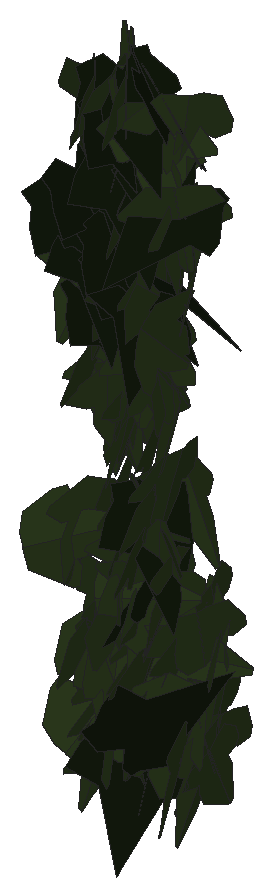
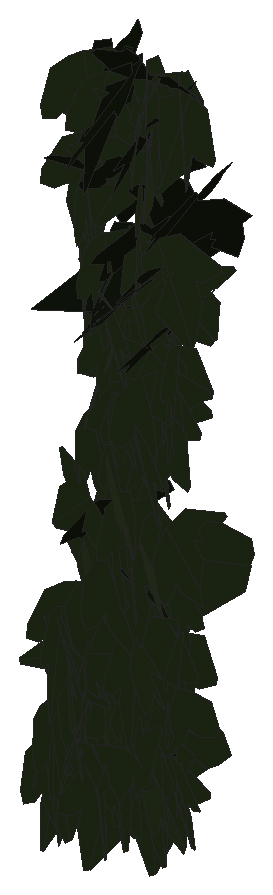
# SketchUp Ruby script. Lengths in inches.
U = 1.inch
M = Sketchup.active_model
def pt(a) = Geom::Point3d.new(a.map { |v| v * U })
def face(e, loops, mat)
  f = e.add_face(loops[0].map { |a| pt(a) })
  loops[1..].each { |l| e.add_face(l.map { |a| pt(a) }).erase! }
  f.material = f.back_material = mat if mat
  f
end
# faces: each face lists its corners as indices into pts; further lists are holes
def faces(e, pts, list, mat = nil) = list.each { |f| face(e, (f[0].is_a?(Array) ? f : [f]).map { |l| l.map { |i| pts[i] } }, mat) }
# xy, xz, yz: faces in a plane at the given z, y or x. An outline is a flat list of corners, or four numbers for a rectangle; further outlines are holes
def ring(l) = l.size == 4 ? [[l[0], l[1]], [l[2], l[1]], [l[2], l[3]], [l[0], l[3]]] : l.each_slice(2).to_a
def flat(e, list, mat, &to3) = list.each { |f| face(e, (f[0].is_a?(Array) ? f : [f]).map { |l| ring(l).map { |u, v| to3.(u, v) } }, mat) }
def xy(e, z, list, mat = nil) = flat(e, list, mat) { |x, y| [x, y, z] }
def xz(e, y, list, mat = nil) = flat(e, list, mat) { |x, z| [x, y, z] }
def yz(e, x, list, mat = nil) = flat(e, list, mat) { |y, z| [x, y, z] }
def lines(e, pts, list) = list.each { |a, b| e.add_line(pt(pts[a]), pt(pts[b])) }
# prism: a flat outline (further loops are holes) pulled along v
def prism(e, loops, v, mat = nil)
  f = face(e, loops, mat); d = Geom::Vector3d.new(v.map { |x| x * U })
  f.pushpull(f.normal.samedirection?(d) ? d.length : -d.length)
end
def box(e, o, s, mat = nil) = prism(e, [[o, [o[0] + s[0], o[1], o[2]], [o[0] + s[0], o[1] + s[1], o[2]], [o[0], o[1] + s[1], o[2]]]], [0, 0, s[2]], mat)
def at(x, y, z, deg = 0) = Geom::Transformation.translation(pt([x, y, z])) * Geom::Transformation.rotation(ORIGIN, Z_AXIS, deg.degrees)
def axes(o, x, y, z) = Geom::Transformation.new([*x, 0, *y, 0, *z, 0, *pt(o).to_a, 1])
def part(name) = M.definitions.add(name)
# library, detail: a bought-in or finely detailed component or shape, given as its bounding box
def library(name, o, s) = part(name).tap { |d| box(d.entities, o, s) }
def detail(e, o, s) = box(e.add_group.entities, o, s)
def put(e, d, t, mat = nil) = e.add_instance(d, t).tap { |i| i.material = mat if mat }
def group(e, t, mat = nil) = e.add_group.tap { |g| g.transformation = t; g.material = mat if mat }.entities
root = M.entities
M.materials.add("efeu1").color = [18, 25, 13]
M.materials.add("efeu2").color = [43, 57, 29]
c1 = part("ivyleaf_10")
p = [[0,0.5,-0.03],[-0.0625,2.02,-0.43],[-0.19,2.01,-0.46],[-0.54,1.05,-0.29],[-0.52,0.625,-0.18],[-0.83,0.76,-0.28],
  [-1.16,0.64,-0.33],[-1.15,0.33,-0.24],[-0.77,-0.39,0.02],[-0.3,-0.51,0.16],[0.04,-0.48,0.23],[-0.02,2.01,-0.4375],
  [-0.06,2.01,-0.43],[0.04,-0.49,0.23],[0.67,-0.49,0.14],[1.38,0.36,-0.2],[1.375,0.51,-0.24],[0.81,0.65,-0.19],
  [0.62,0.59,-0.15],[0.6,1.09,-0.28],[0.5,1.23,-0.31]]
faces(c1.entities,p,[[0,1,2,3,4,5,6,7,8,9,10],[11,12,0,13,14,15,16,17,18,19,20]],"efeu2")
c2 = part("ivyleaf_9")
p = [[1.54,2.16,1.25],[1.36,2.04,1.19],[-0.21,0.99,0.68],[-0.71,1.11,0.82],[-0.85,0.86,0.67],[-0.8,0.17,0.21],
  [-0.9,-0.01,0.1],[-0.67,-0.16,-0.02],[-0.08,-0.08,-0.05],[-0.03,-0.6,-0.4],[0.65,-0.88,-0.66],[0.83,-0.6,-0.49],
  [1.29,-0.42,-0.43],[1.8125,-0.07,-0.26],[1.21,0.44,0.15]]
faces(c2.entities,p,[[0,1,2,3,4,5,6,7,8,9,10,11,12,13,14]],"efeu1")
put(root,c1,axes([19.25,224.81,220.86],[-0.42384,-0.16044,0.21122],[-0.18486,-0.10687,-0.45211],[0.19022,-0.46134,0.03127]))
put(root,c1,axes([19.05,224.78,217.3],[-0.02524,-0.43944,0.23719],[0.06704,-0.23832,-0.43441],[0.49484,0.00987,0.07095]))
put(root,c1,axes([19.06,225.11,214.47],[0.12032,-0.4664,0.13412],[0.03183,-0.1303,-0.48167],[0.48426,0.12445,-0.00167]))
put(root,c1,axes([18.77,224.23,216.92],[0.07583,0.04521,-0.49214],[0.42938,0.2405,0.08825],[0.2447,-0.43602,-0.00235]))
put(root,c1,axes([19.11,224.54,215.75],[0.05155,-0.43916,-0.23342],[0.04918,0.23802,-0.43695],[0.4949,0.02209,0.06774]))
put(root,c1,axes([19.14,224.71,220.44],[-0.21372,-0.34408,0.29314],[0.05065,-0.34044,-0.36267],[0.44918,-0.12532,0.18037]))
put(root,c1,axes([19.35,224.875,214.3],[-0.36082,0.16197,0.30589],[-0.29662,0.08304,-0.39385],[-0.17839,-0.46569,0.03616]))
put(root,c1,axes([19.12,224.66,222.71],[-0.4928,0.05479,-0.06441],[0.06274,-0.01843,-0.49571],[-0.0567,-0.49665,0.01129]))
put(root,c1,axes([18.9375,224.98,215.45],[0.43453,0.18103,0.16855],[0.15335,0.07018,-0.4707],[-0.19408,0.46076,0.00546]))
put(root,c1,axes([19.1875,224.95,214.75],[-0.00417,-0.49987,-0.01051],[0.00087,0.0105,-0.49989],[0.49998,-0.00419,0.00078]))
put(root,c1,axes([19.2,224.53,219.39],[0.04854,-0.43156,-0.24778],[-0.01141,0.24793,-0.43405],[0.49751,0.04779,0.01422]))
put(root,c1,axes([19.2,225.08,215.99],[0.07684,-0.45309,0.19698],[0.02088,-0.19619,-0.45943],[0.49362,0.07883,-0.01123]))
put(root,c1,axes([19.22,224.67,214.375],[0.39934,-0.29803,-0.04127],[-0.0295,0.02947,-0.49826],[0.29942,0.40039,0.00595]))
put(root,c1,axes([19.24,224.42,222.76],[0.21719,-0.434,-0.12029],[0.00579,0.13623,-0.48105],[0.45033,0.20756,0.0642]))
put(root,c1,axes([19.28,224.93,214.23],[-0.18051,-0.46447,-0.04109],[0.00929,0.04047,-0.49827],[0.46619,-0.18065,-0.00599]))
put(root,c1,axes([19.1,225.21,217.36],[0.24568,-0.33864,0.2738],[0.18002,-0.20727,-0.41789],[0.39653,0.30391,0.02008]))
put(root,c1,axes([19.19,224.91,218.74],[-0.46671,0.09561,-0.1518],[0.13308,-0.09922,-0.47164],[-0.12031,-0.48064,0.06717]))
put(root,c2,axes([19.05,224.47,221.6],[0.26423,-0.36255,-0.22078],[-0.06525,0.22228,-0.4431],[0.41943,0.26297,0.07015]))
put(root,c1,axes([19.07,224.47,214.43],[0.3595,0.16802,-0.30419],[0.24594,0.18619,0.3935],[0.24551,-0.43255,0.05122]))
put(root,c1,axes([19.06,225.5,214.69],[-0.29912,0.08817,0.39084],[0.35602,-0.16523,0.30975],[0.18378,0.4636,0.03607]))
put(root,c1,axes([19.35,224.93,219.13],[-0.2172,-0.43542,0.11505],[0.01154,-0.13307,-0.48183],[0.45021,-0.20665,0.06786]))
put(root,c1,axes([19.35,224.91,215.25],[-0.1532,-0.46121,-0.11753],[0.043,0.10955,-0.48595],[0.474,-0.159,0.0061]))
put(root,c1,axes([19.375,225.07,215.9],[-0.09383,-0.47191,-0.13601],[0.01906,0.13487,-0.48109],[0.49075,-0.09547,-0.00732]))
put(root,c1,axes([19.48,224.7,222.17],[0.08347,-0.19617,-0.45227],[-0.15164,0.42625,-0.21287],[0.46908,0.1727,0.01166]))
put(root,c2,axes([19.11,224.38,221.47],[-0.07818,-0.25213,-0.42464],[0.25076,0.35011,-0.25405],[0.42545,-0.25268,0.07171]))
put(root,c1,axes([19.47,225.3,214.65],[0.35172,-0.22309,-0.27664],[-0.13015,0.28131,-0.39233],[0.33069,0.34799,0.13981]))
put(root,c1,axes([19.42,224.43,216.42],[0.42925,-0.20419,-0.15508],[-0.08846,0.16591,-0.4633],[0.24066,0.42518,0.10631]))
put(root,c1,axes([19.37,225.03,218.61],[0.37234,-0.33349,-0.01198],[0.00318,0.02149,-0.49953],[0.33369,0.37191,0.01812]))
put(root,c1,axes([19.43,225.62,214.78],[0.48445,-0.00567,-0.12361],[-0.1236,0.00091,-0.48448],[0.00572,0.49997,-0.00052]))
put(root,c1,axes([19.42,224.55,222.79],[0.01604,-0.47537,-0.15416],[0.03051,0.15489,-0.47443],[0.49881,0.00581,0.03398]))
put(root,c1,axes([19.58,224.78,222.38],[-0.1151,0.32188,-0.36489],[-0.13528,0.33901,0.34172],[0.46739,0.17739,0.00905]))
put(root,c1,axes([19.49,225.37,217.01],[-0.13106,-0.46805,0.11726],[-0.01146,-0.11845,-0.48563],[0.48238,-0.12998,0.02032]))
put(root,c1,axes([19.56,224.78,222.43],[-0.15526,0.39744,-0.26065],[-0.09886,0.2412,0.42667],[0.46489,0.18403,0.00369]))
put(root,c1,axes([19.51,224.73,218.94],[-0.30349,-0.39631,0.02883],[-0.01527,-0.02462,-0.49916],[0.39707,-0.30386,0.00284]))
put(root,c2,axes([19.27,224.68,220.74],[-0.01087,-0.49745,-0.0492],[0.00784,0.04904,-0.49753],[0.49982,-0.01159,0.00673]))
put(root,c2,axes([19.2,224.72,220.01],[0.18998,-0.44437,-0.12823],[0.00967,0.14242,-0.47919],[0.4624,0.17959,0.06271]))
put(root,c1,axes([19.48,224.85,218.99],[-0.4196,-0.26374,-0.0662],[0.04786,0.04818,-0.49537],[0.26767,-0.42204,-0.01519]))
put(root,c1,axes([19.61,224.49,218.6],[0.21994,-0.32245,-0.3125],[-0.17437,0.25933,-0.39031],[0.41379,0.28067,0.00162]))
put(root,c1,axes([19.5,224.99,215.09],[0.133,-0.43935,-0.1982],[0.00537,0.20694,-0.45513],[0.48196,0.11893,0.05977]))
put(root,c1,axes([19.63,225.2,214.66],[-0.19161,-0.24676,-0.39038],[-0.24816,-0.30143,0.31234],[-0.38949,0.31345,-0.00695]))
put(root,c1,axes([19.54,225.01,215.27],[-0.23432,-0.4391,-0.04777],[0.02052,0.0432,-0.49771],[0.44122,-0.23521,-0.00222]))
put(root,c1,axes([19.54,224.7,215.85],[-0.49109,-0.09296,-0.01357],[0.01354,0.00142,-0.49981],[0.09297,-0.49128,0.00112]))
put(root,c1,axes([19.66,225.4,214.47],[0.20499,-0.27668,-0.36252],[-0.16336,0.32654,-0.34159],[0.42578,0.25849,0.04348]))
put(root,c1,axes([19.56,225.09,215.37],[0.05916,-0.49644,0.00679],[0.00057,-0.00677,-0.49995],[0.49649,0.05916,-0.00024]))
put(root,c1,axes([19.57,225.01,217.56],[-0.06786,-0.48411,-0.10502],[0.01704,0.10366,-0.48884],[0.49508,-0.06993,0.00243]))
put(root,c1,axes([19.53,224.67,220.38],[0.10224,-0.45221,0.18722],[0.04689,-0.18133,-0.4636],[0.48718,0.11235,0.00533]))
put(root,c1,axes([19.47,224.63,215.54],[0.10552,0.48835,-0.0195],[-0.00424,-0.01904,-0.49962],[-0.48872,0.10561,0.00012]))
put(root,c1,axes([19.53,225.38,214.35],[-0.29759,-0.38523,-0.11419],[0.11036,0.05827,-0.48418],[0.38634,-0.31338,0.05034]))
put(root,c1,axes([19.5,224.62,215.54],[0.21026,0.43828,-0.11706],[-0.04571,-0.1079,-0.48607],[-0.45133,0.21511,-0.0053]))
put(root,c1,axes([19.56,225.23,218.19],[0.23365,-0.44124,0.02679],[0.02251,-0.01839,-0.49915],[0.44148,0.23446,0.01127]))
put(root,c1,axes([19.62,224.77,217.27],[0.1273,-0.4384,-0.20396],[-0.03483,0.20205,-0.45603],[0.48227,0.13032,0.0209]))
put(root,c1,axes([19.61,224.65,221.44],[0.14527,-0.41065,-0.24548],[-0.01493,0.25253,-0.43128],[0.4782,0.13264,0.06111]))
put(root,c1,axes([19.625,224.94,218.89],[0.06465,-0.48744,0.09069],[-0.00171,-0.09167,-0.49152],[0.4958,0.06324,-0.01352]))
put(root,c2,axes([19.52,224.96,214.17],[-0.13531,-0.48128,-0.00798],[0.00114,0.00797,-0.49994],[0.48134,-0.13531,-0.00106]))
put(root,c1,axes([19.6,225.36,215.96],[-0.03222,-0.17268,0.46813],[0.07971,-0.46486,-0.16598],[0.49255,0.06393,0.05748]))
put(root,c2,axes([19.4375,224.62,222.51],[0.21858,-0.40541,-0.19458],[-0.09207,0.17142,-0.46059],[0.44016,0.23718,0.00029]))
put(root,c1,axes([19.64,224.51,222.86],[0.19746,-0.43702,-0.14149],[0.0234,0.16338,-0.47197],[0.45876,0.17977,0.08497]))
put(root,c1,axes([19.59,224.8125,219.38],[-0.47327,0.03073,-0.15835],[0.15529,-0.04603,-0.47304],[-0.04365,-0.49693,0.03402]))
put(root,c1,axes([19.97,224.67,214.62],[0.26087,-0.01404,-0.42632],[-0.40348,0.154,-0.25197],[0.13838,0.47549,0.06901]))
put(root,c1,axes([19.68,224.65,222.78],[0.49646,0.03244,-0.04974],[-0.04935,-0.00767,-0.4975],[-0.03304,0.49889,-0.00441]))
put(root,c1,axes([19.38,225.18,214.71],[-0.17867,0.0609,-0.463],[0.429,-0.17445,-0.18849],[-0.18449,-0.46461,0.01009]))
put(root,c2,axes([19.45,224.75,220.52],[0.25041,-0.39789,-0.17024],[0.03279,0.21356,-0.45091],[0.43153,0.21466,0.13305]))
put(root,c2,axes([19.92,224.28,216.38],[-0.39021,0.26144,-0.17142],[-0.14436,0.0925,0.46968],[0.2773,0.41604,0.0033]))
put(root,c1,axes([20.01,224.42,219.41],[-0.40358,-0.00296,0.29516],[-0.29331,-0.05212,-0.40157],[0.03314,-0.49727,0.04033]))
put(root,c1,axes([19.89,224.65,214.38],[0.18192,-0.28461,-0.36865],[-0.14185,0.34311,-0.33489],[0.4436,0.22643,0.0441]))
put(root,c1,axes([19.85,224.67,219.54],[-0.46813,-0.16766,0.05237],[-0.01811,-0.10223,-0.4891],[0.17471,-0.45982,0.08965]))
put(root,c2,axes([19.58,224.61,221.04],[0.11577,-0.39214,-0.28779],[-0.0177,0.29224,-0.40532],[0.48609,0.10403,0.05379]))
put(root,c1,axes([19.72,224.18,216.33],[-0.04587,-0.24938,-0.43094],[0.15736,0.40332,-0.25014],[0.47237,-0.15857,0.04148]))
put(root,c1,axes([19.87,225.4,215.42],[-0.05341,-0.46814,0.16732],[-0.0077,-0.16748,-0.47105],[0.49708,-0.05289,0.01068]))
put(root,c1,axes([19.96,224.625,217.07],[-0.34038,-0.33892,0.13885],[-0.07858,-0.11756,-0.47959],[0.35773,-0.3483,0.02677]))
put(root,c2,axes([19.6,224.59,223.01],[-0.17637,-0.24166,-0.40062],[0.36755,0.19334,-0.27844],[0.28949,-0.39271,0.10944]))
put(root,c2,axes([19.7,224.66,221.91],[-0.09932,-0.45644,-0.17833],[0.07791,0.16493,-0.46554],[0.4838,-0.12026,0.03836]))
put(root,c1,axes([19.84,224.95,215.02],[0.16906,-0.41563,0.22062],[0.07076,-0.2093,-0.44854],[0.4652,0.18288,-0.01195]))
put(root,c1,axes([19.91,224.63,215.62],[0.09597,-0.48946,0.03486],[0.00162,-0.0352,-0.49876],[0.4907,0.09585,-0.00517]))
put(root,c1,axes([19.89,224.72,216.22],[0.32997,-0.37316,-0.04329],[-0.02668,0.0342,-0.49811],[0.37471,0.33103,0.00266]))
put(root,c1,axes([19.91,224.86,215.01],[0.01122,-0.45,0.21766],[0.02439,-0.21697,-0.44981],[0.49928,0.02071,0.01708]))
put(root,c1,axes([19.77,224.9375,216.32],[-0.01318,-0.04921,0.4974],[0.24444,-0.43465,-0.03653],[0.43598,0.2422,0.03551]))
put(root,c1,axes([19.91,224.96,220.09],[0.37016,-0.33452,-0.03281],[-0.01763,0.02942,-0.49882],[0.33567,0.37044,0.00998]))
put(root,c1,axes([19.99,224.38,217.29],[0.15677,-0.43403,-0.19247],[-0.04614,0.1878,-0.46109],[0.47254,0.16233,0.01883]))
put(root,c1,axes([19.91,224.73,219.7],[-0.16867,-0.46775,-0.05258],[0.10945,0.01535,-0.48763],[0.45779,-0.176,0.09721]))
put(root,c1,axes([19.99,225.05,215.56],[0.06373,-0.4011,-0.29165],[-0.02222,0.29144,-0.40567],[0.49542,0.06467,0.01932]))
put(root,c1,axes([19.99,225.39,215.4],[0.16368,-0.4513,-0.13977],[-0.02676,0.13883,-0.47959],[0.47169,0.16448,0.02129]))
put(root,c1,axes([20.07,224.92,216.36],[-0.19357,-0.36727,0.27864],[-0.04569,-0.28544,-0.40797],[0.45874,-0.1834,0.07694]))
put(root,c2,axes([19.82,224.76,220.23],[-0.04788,-0.47793,0.13889],[0.02054,-0.14131,-0.47918],[0.49728,-0.04019,0.03316]))
put(root,c1,axes([20.18,224.6,217.02],[-0.40549,0.20361,-0.21004],[-0.18991,0.08985,0.45372],[0.22251,0.44774,0.00447]))
put(root,c1,axes([19.76,224.7,221.91],[0.3626,0.26158,0.22383],[0.17584,0.13877,-0.44702],[-0.29598,0.40289,0.00864]))
put(root,c1,axes([20.05,224.61,222.63],[-0.35073,-0.35619,-0.01078],[0.00983,0.00545,-0.49987],[0.35622,-0.35085,0.00318]))
put(root,c1,axes([20.36,225.3,215.71],[-0.05275,0.09799,0.48746],[-0.49503,0.03548,-0.0607],[-0.04649,-0.48902,0.09327]))
put(root,c1,axes([20.04,224.78,220.64],[-0.05649,-0.48881,-0.08873],[0.02179,0.08678,-0.49193],[0.49632,-0.05944,0.0115]))
put(root,c1,axes([20.02,224.99,215.25],[-0.08763,-0.40452,-0.2805],[0.06669,0.27253,-0.41386],[0.48772,-0.10994,0.00619]))
put(root,c2,axes([19.9,224.57,223.08],[0.40192,-0.17477,-0.24066],[-0.20707,0.12599,-0.43732],[0.2135,0.4512,0.0289]))
put(root,c1,axes([20.02,224.4,220.52],[0.05536,-0.3212,-0.37917],[0.07246,0.38265,-0.31357],[0.49162,-0.02023,0.08891]))
put(root,c1,axes([20.03,225.32,214.95],[-0.28165,0.41285,0.01493],[-0.00831,0.0124,-0.49978],[-0.41304,-0.28178,-0.00012]))
put(root,c1,axes([20.12,225.05,214.84],[0.43225,-0.20576,-0.1443],[-0.12289,0.07736,-0.47845],[0.21922,0.44909,0.01631]))
put(root,c1,axes([19.68,224.39,216.4375],[0.09266,-0.0787,-0.485],[0.49133,0.01264,0.09182],[-0.00219,-0.49361,0.07967]))
put(root,c2,axes([20.16,224.56,222.93],[0.33162,0.04646,-0.37131],[-0.37361,0.06908,-0.32503],[0.0211,0.49302,0.08053]))
put(root,c2,axes([19.74,224.81,220.58],[0.41197,-0.27593,0.06434],[0.10984,0.05088,-0.48513],[0.26118,0.41385,0.10254]))
put(root,c2,axes([19.94,224.76,217.54],[0.00545,-0.48353,-0.12716],[-0.01178,0.12701,-0.48346],[0.49983,0.00827,-0.01]))
put(root,c1,axes([20.1,224.5625,216.62],[-0.4565,-0.20171,0.03034],[0.02777,0.01222,0.49908],[-0.20208,0.45734,0.00005]))
put(root,c1,axes([20.22,224.84,215.1],[-0.20692,-0.36173,0.27629],[-0.06206,-0.27825,-0.41076],[0.45093,-0.20428,0.07025]))
put(root,c1,axes([19.8,224.66,222.2],[0.35766,-0.00956,0.34927],[0.34722,0.06544,-0.35377],[-0.03895,0.49561,0.05345]))
put(root,c1,axes([20.15,225.45,216.13],[0.05675,-0.45527,-0.19878],[0.02875,0.20275,-0.45614],[0.49594,0.04034,0.04919]))
put(root,c1,axes([20.16,225.05,215.75],[0.10179,-0.4805,0.09358],[0.01057,-0.0934,-0.49109],[0.48942,0.10195,-0.00885]))
put(root,c1,axes([20.18,224.38,217.9],[0.03947,-0.43582,-0.24187],[0.00032,0.24265,-0.43717],[0.49844,0.03436,0.01944]))
put(root,c1,axes([20.14,224.55,219.43],[0.2268,-0.337,-0.29153],[0.05375,0.34542,-0.35748],[0.44235,0.13082,0.19291]))
put(root,c1,axes([20.0625,224.63,222.47],[0.45298,0.2047,0.0539],[0.04675,0.02743,-0.49705],[-0.20645,0.45535,0.00571]))
put(root,c1,axes([20.26,225.4375,214.49],[-0.14025,-0.47861,0.03558],[-0.01413,-0.03293,-0.49871],[0.47972,-0.14089,-0.00429]))
put(root,c2,axes([19.94,224.25,214.6875],[0.01116,-0.05102,0.49727],[0.46967,0.17134,0.00704],[-0.17112,0.46695,0.05175]))
put(root,c1,axes([20.28,225.45,214.89],[0.04068,-0.49636,-0.04445],[-0.00601,0.04411,-0.49801],[0.49831,0.04106,-0.00238]))
put(root,c1,axes([20.2,224.79,216.81],[0.17341,-0.39374,0.25475],[0.10017,-0.23425,-0.43023],[0.45814,0.20025,-0.00236]))
put(root,c1,axes([20.31,224.62,218.25],[0.01401,-0.49933,0.02169],[-0.00312,-0.02179,-0.49952],[0.49979,0.01387,-0.00373]))
put(root,c1,axes([20.27,225.35,214.46],[0.1481,-0.4655,-0.10667],[0.02689,0.11964,-0.48473],[0.47681,0.13784,0.06047]))
put(root,c2,axes([20.41,224.75,221.74],[-0.42826,-0.25259,0.05284],[-0.03454,-0.04535,-0.49674],[0.25573,-0.42912,0.02139]))
put(root,c1,axes([19.98,224.8,215.66],[0.04324,0.06516,0.49385],[0.34052,0.35793,-0.07704],[-0.36356,0.34299,-0.01342]))
put(root,c1,axes([20.35,224.49,218.92],[0.31108,-0.38403,-0.07585],[-0.03628,0.06818,-0.494],[0.38976,0.31285,0.01455]))
put(root,c1,axes([20.28,224.8,221.42],[0.10613,-0.48394,0.06735],[0.11452,-0.04236,-0.48486],[0.475,0.11834,0.10185]))
put(root,c1,axes([20.48,224.68,220.75],[0.15963,-0.26136,-0.39523],[-0.16329,0.36117,-0.30479],[0.44481,0.22638,0.02995]))
put(root,c1,axes([20.34,225.22,215.75],[0.36457,-0.34185,-0.01501],[-0.00642,0.0151,-0.49973],[0.34212,0.36457,0.00663]))
put(root,c1,axes([20.43,224.6875,222.79],[-0.2989,-0.39572,0.06372],[-0.00428,-0.07633,-0.49412],[0.4008,-0.29593,0.04225]))
put(root,c1,axes([20.39,225.16,214.26],[-0.02078,-0.42867,-0.25653],[0.02395,0.2556,-0.42906],[0.49899,-0.03012,0.00991]))
put(root,c1,axes([20.41,224.11,220.13],[0.00988,0.3257,0.37924],[-0.15475,0.36268,-0.30744],[-0.47535,-0.1113,0.10797]))
put(root,c1,axes([20.04,225.16,217.67],[0.29896,-0.07958,0.39279],[0.38995,-0.05539,-0.30802],[0.09254,0.49051,0.02895]))
put(root,c1,axes([20.28,225.1875,214.21],[0.05923,-0.36899,0.33218],[0.16348,-0.30138,-0.36393],[0.46879,0.15172,0.08494]))
put(root,c1,axes([20.25,224.79,214.52],[0.23396,-0.31948,0.30528],[0.18569,-0.24237,-0.39595],[0.40098,0.29865,0.00523]))
put(root,c1,axes([20.42,224.53,221.69],[-0.40101,-0.29577,-0.04134],[0.03576,0.02116,-0.49827],[0.2965,-0.40258,0.00418]))
put(root,c1,axes([20.42,224.9,216.11],[-0.25642,-0.41992,-0.08895],[0.03916,0.08029,-0.49195],[0.42745,-0.25926,-0.00829]))
